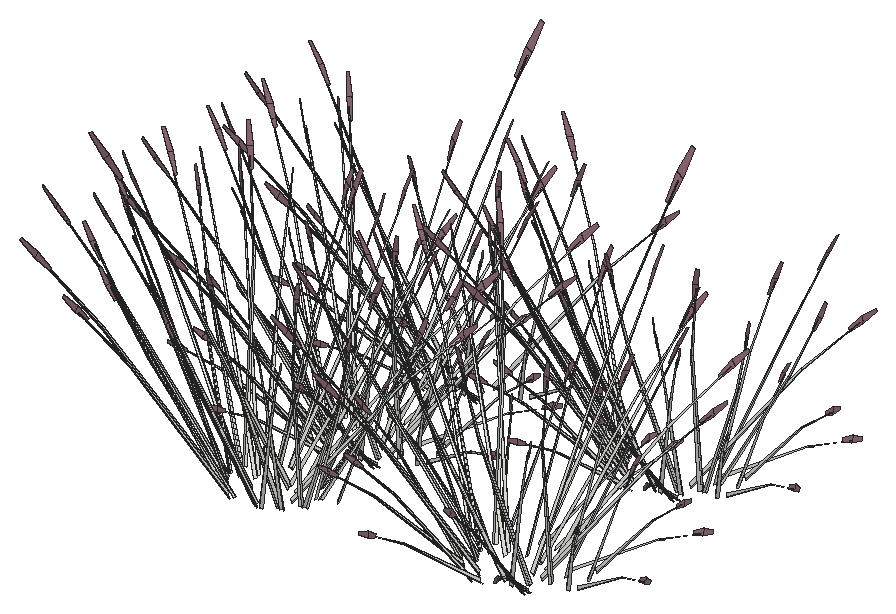
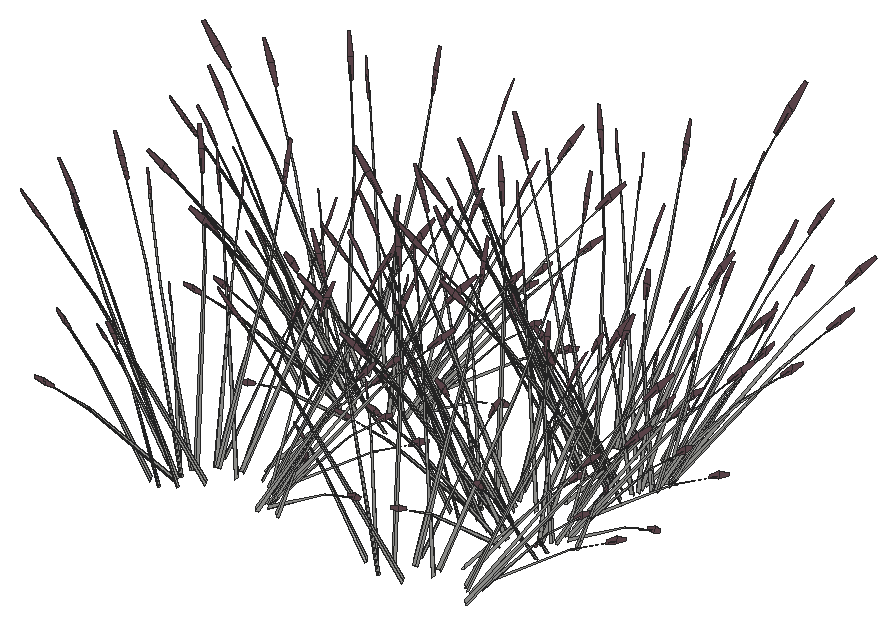
# SketchUp Ruby script. Lengths in inches.
U = 1.inch
M = Sketchup.active_model
def pt(a) = Geom::Point3d.new(a.map { |v| v * U })
def face(e, loops, mat)
  f = e.add_face(loops[0].map { |a| pt(a) })
  loops[1..].each { |l| e.add_face(l.map { |a| pt(a) }).erase! }
  f.material = f.back_material = mat if mat
  f
end
# faces: each face lists its corners as indices into pts; further lists are holes
def faces(e, pts, list, mat = nil) = list.each { |f| face(e, (f[0].is_a?(Array) ? f : [f]).map { |l| l.map { |i| pts[i] } }, mat) }
# xy, xz, yz: faces in a plane at the given z, y or x. An outline is a flat list of corners, or four numbers for a rectangle; further outlines are holes
def ring(l) = l.size == 4 ? [[l[0], l[1]], [l[2], l[1]], [l[2], l[3]], [l[0], l[3]]] : l.each_slice(2).to_a
def flat(e, list, mat, &to3) = list.each { |f| face(e, (f[0].is_a?(Array) ? f : [f]).map { |l| ring(l).map { |u, v| to3.(u, v) } }, mat) }
def xy(e, z, list, mat = nil) = flat(e, list, mat) { |x, y| [x, y, z] }
def xz(e, y, list, mat = nil) = flat(e, list, mat) { |x, z| [x, y, z] }
def yz(e, x, list, mat = nil) = flat(e, list, mat) { |y, z| [x, y, z] }
def lines(e, pts, list) = list.each { |a, b| e.add_line(pt(pts[a]), pt(pts[b])) }
# prism: a flat outline (further loops are holes) pulled along v
def prism(e, loops, v, mat = nil)
  f = face(e, loops, mat); d = Geom::Vector3d.new(v.map { |x| x * U })
  f.pushpull(f.normal.samedirection?(d) ? d.length : -d.length)
end
def box(e, o, s, mat = nil) = prism(e, [[o, [o[0] + s[0], o[1], o[2]], [o[0] + s[0], o[1] + s[1], o[2]], [o[0], o[1] + s[1], o[2]]]], [0, 0, s[2]], mat)
def at(x, y, z, deg = 0) = Geom::Transformation.translation(pt([x, y, z])) * Geom::Transformation.rotation(ORIGIN, Z_AXIS, deg.degrees)
def axes(o, x, y, z) = Geom::Transformation.new([*x, 0, *y, 0, *z, 0, *pt(o).to_a, 1])
def part(name) = M.definitions.add(name)
# library, detail: a bought-in or finely detailed component or shape, given as its bounding box
def library(name, o, s) = part(name).tap { |d| box(d.entities, o, s) }
def detail(e, o, s) = box(e.add_group.entities, o, s)
def put(e, d, t, mat = nil) = e.add_instance(d, t).tap { |i| i.material = mat if mat }
def group(e, t, mat = nil) = e.add_group.tap { |g| g.transformation = t; g.material = mat if mat }.entities
root = M.entities
M.materials.add("LightPink_Translucent").color = [144, 107, 117]
c1 = part("blade")
p = [[2.15,0.21,22],[0,0.17,0],[0.09,0.45,0],[2.18,0.31,22],[2.29,0.31,22],[0.38,0.45,0],
  [2.48,0.24,33],[2.49,0.24,33],[2.48,0.22,33]]
faces(c1.entities,p,[[0,1,2,3],[4,5,2,3],[6,3,4,7],[8,0,3,6]])
c2 = part("seeds")
p = [[0.3,-0.1,1.38],[-0.01,-0.03,1.59],[-0.01,-0.03,0.03],[0.14,-0.07,-0.07],[0.29,-0.03,3],[0.15,0.01,3.11]]
faces(c2.entities,p,[[0,1,2,3],[1,0,4,5]],"LightPink_Translucent")
c3 = part("blade with seeds")
put(c3.entities,c1,at(0,0,0))
put(c3.entities,c2,axes([2.4,0.25,30.99],[1.5799,-0.05474,1.17369],[-0.12525,1.92788,0.29478],[-0.07173,-0.02425,1.56792]))
put(root,c3,axes([27.78,17.96,46.13],[0.28013,0.33252,1.71376],[-1.29445,0.27994,0.13857],[-0.29256,-0.52202,0.73262]))
put(root,c3,axes([31.34,17.49,46.78],[0.36946,-0.79643,-0.35414],[1.07787,0.23229,0.4572],[-0.09883,-0.32066,0.87481]))
put(root,c3,axes([32.15,18.55,46.13],[-0.22818,0.35597,1.71376],[-0.95725,-0.73667,0.13857],[0.43183,-0.45914,0.73262]))
put(root,c3,axes([31.82,18,47.29],[-1.19922,0.48218,-0.1216],[-0.58932,-0.85579,-0.67495],[-0.15822,-0.36063,1.02557]))
put(root,c3,axes([34.3125,19.08,47.29],[-1.34686,-0.05131,-0.1216],[0.03681,-0.97156,-0.67495],[0.09356,-0.37418,1.02557]))
put(root,c3,axes([34.22,18.46,46.78],[0.82919,-0.54528,-0.35414],[0.78493,0.62262,0.4572],[0.11943,-0.31634,0.87481]))
put(root,c3,axes([28.23,17.78,46.78],[-0.18927,-0.83419,-0.35414],[1.08199,-0.22027,0.4572],[-0.29062,-0.23905,0.87481]))
put(root,c3,axes([60.8,22.02,45.875],[0.28013,0.33252,1.71376],[-1.29445,0.27994,0.13857],[-0.29256,-0.52202,0.73262]))
put(root,c3,axes([25.9,19,46.13],[0.45521,0.17844,1.71376],[-0.94204,0.74856,0.13857],[-0.58713,-0.33769,0.73262]))
put(root,c3,axes([62.93,19.82,46.72],[-0.18744,-0.14521,1.74944],[-1.25089,0.09206,-0.27667],[-0.19964,-0.34731,0.14031]))
put(root,c3,axes([68.55,21.6,46.72],[-0.01183,-0.20612,1.74944],[-0.99913,-0.59572,-0.27667],[0.15447,-0.36112,0.14031]))
put(root,c3,axes([65.17,22.61,45.875],[-0.22818,0.35597,1.71376],[-0.95725,-0.73667,0.13857],[0.43183,-0.45914,0.73262]))
put(root,c3,axes([68.29,20.86,46.71],[-0.12446,0.07911,1.77383],[-1.21937,-0.26689,-0.16761],[-0.04414,-0.34521,0.31391]))
put(root,c3,axes([35.78,20.99,47.29],[-1.1336,-0.57106,-0.1216],[0.65308,-0.827,-0.67495],[0.32027,-0.28747,1.02557]))
put(root,c3,axes([31.1,24.11,45.58],[1.05902,0.41762,1.51261],[-1.03748,0.89969,0.59816],[-0.46471,-0.53324,1.26806]))
put(root,c3,axes([61.65,19.34,46.71],[-0.02286,0.12414,1.77383],[-1.12758,0.45052,-0.16761],[-0.33182,-0.23029,0.31391]))
put(root,c3,axes([64.84,22.06,47.03],[-1.19922,0.48218,-0.1216],[-0.58932,-0.85579,-0.67495],[-0.15822,-0.36063,1.02557]))
put(root,c3,axes([67.33,23.14,47.03],[-1.34686,-0.05131,-0.1216],[0.03681,-0.97156,-0.67495],[0.09356,-0.37418,1.02557]))
put(root,c3,axes([36.1,20.41,46.78],[1.06674,-0.14801,-0.35414],[0.28168,0.84611,0.4572],[0.30569,-0.22726,0.87481]))
put(root,c3,axes([25.73,19.25,46.78],[-0.69728,-0.64842,-0.35414],[0.79619,-0.61382,0.4572],[-0.40453,-0.09339,0.87481]))
put(root,c3,axes([58.92,23.06,45.875],[0.45521,0.17844,1.71376],[-0.94204,0.74856,0.13857],[-0.58713,-0.33769,0.73262]))
put(root,c3,axes([58.83,21.41,46.72],[-0.26368,-0.00731,1.74944],[-0.83946,0.73103,-0.27667],[-0.44791,-0.14937,0.14031]))
put(root,c3,axes([68.79,25.05,47.03],[-1.1336,-0.57106,-0.1216],[0.65308,-0.827,-0.67495],[0.32027,-0.28747,1.02557]))
put(root,c3,axes([26.53,19.18,47.29],[-0.06562,1.05324,-0.1216],[-1.2424,-0.02879,-0.67495],[-0.4785,-0.07316,1.02557]))
put(root,c3,axes([35.82,23.22,47.29],[-0.6166,-0.93779,-0.1216],[1.09436,-0.46085,-0.67495],[0.46117,-0.12373,1.02557]))
put(root,c3,axes([71.59,24.8,46.71],[-0.16006,-0.00787,1.77383],[-0.66468,-0.8428,-0.16761],[0.26693,-0.27711,0.31391]))
put(root,c3,axes([24.94,20.63,46.13],[0.50831,-0.02346,1.71376],[-0.33721,1.01661,0.13857],[-0.72439,-0.06288,0.73262]))
put(root,c3,axes([36.47,22.84,46.78],[1.01846,0.28891,-0.35414],[-0.29705,0.84289,0.4572],[0.41005,-0.07729,0.87481]))
put(root,c3,axes([72.1875,25.8125,46.72],[0.17006,-0.15775,1.74944],[-0.21766,-0.96766,-0.27667],[0.42669,-0.18347,0.14031]))
put(root,c3,axes([24.5,21.5,46.78],[-1.01846,-0.28891,-0.35414],[0.29705,-0.84289,0.4572],[-0.41005,0.07729,0.87481]))
put(root,c3,axes([57.82,22.03,46.71],[0.09085,0.10335,1.77383],[-0.43798,0.92907,-0.16761],[-0.44357,0.00672,0.31391]))
put(root,c3,axes([33.69,21.8,46.13],[-0.50831,0.02346,1.71376],[0.33721,-1.01661,0.13857],[0.72439,0.06288,0.73262]))
put(root,c3,axes([59.54,23.24,47.03],[-0.06562,1.05324,-0.1216],[-1.2424,-0.02879,-0.67495],[-0.4785,-0.07316,1.02557]))
put(root,c3,axes([68.84,27.28,47.03],[-0.6166,-0.93779,-0.1216],[1.09436,-0.46085,-0.67495],[0.46117,-0.12373,1.02557]))
put(root,c3,axes([57.96,24.69,45.875],[0.50831,-0.02346,1.71376],[-0.33721,1.01661,0.13857],[-0.72439,-0.06288,0.73262]))
put(root,c3,axes([27.6,21.36,45.59],[0.34834,-0.14982,1.77064],[0.12012,1.04605,0.13857],[-0.75452,0.1388,0.63284]))
put(root,c3,axes([25.14,21.125,47.29],[0.6166,0.93779,-0.1216],[-1.09436,0.46085,-0.67495],[-0.46117,0.12373,1.02557]))
put(root,c3,axes([37.3125,25.19,46.18],[-0.23455,-0.87059,-0.03492],[1.10861,-0.20015,-0.15832],[0.23151,0.05519,0.52218]))
put(root,c3,axes([34.4375,25.17,47.29],[0.06562,-1.05324,-0.1216],[1.2424,0.02879,-0.67495],[0.4785,0.07316,1.02557]))
put(root,c3,axes([29.33,34.02,45.875],[0.28013,0.33252,1.71376],[-1.29445,0.27994,0.13857],[-0.29256,-0.52202,0.73262]))
put(root,c3,axes([31.46,31.82,46.72],[-0.18744,-0.14521,1.74944],[-1.25089,0.09206,-0.27667],[-0.19964,-0.34731,0.14031]))
put(root,c3,axes([25.16,22.42,46.13],[0.42521,-0.21906,1.71376],[0.35798,1.01226,0.13857],[-0.66754,0.22878,0.73262]))
put(root,c3,axes([37.08,33.6,46.72],[-0.01183,-0.20612,1.74944],[-0.99913,-0.59572,-0.27667],[0.15447,-0.36112,0.14031]))
put(root,c3,axes([33.7,34.61,45.875],[-0.22818,0.35597,1.71376],[-0.95725,-0.73667,0.13857],[0.43183,-0.45914,0.73262]))
put(root,c3,axes([36.81,32.86,46.71],[-0.12446,0.07911,1.77383],[-1.21937,-0.26689,-0.16761],[-0.04414,-0.34521,0.31391]))
put(root,c3,axes([66.71,25.86,45.875],[-0.50831,0.02346,1.71376],[0.33721,-1.01661,0.13857],[0.72439,0.06288,0.73262]))
put(root,c3,axes([30.18,31.34,46.71],[-0.02286,0.12414,1.77383],[-1.12758,0.45052,-0.16761],[-0.33182,-0.23029,0.31391]))
put(root,c3,axes([35.24,25.1,46.78],[0.69728,0.64842,-0.35414],[-0.79619,0.61382,0.4572],[0.40453,0.09339,0.87481]))
put(root,c3,axes([33.37,34.06,47.03],[-1.19922,0.48218,-0.1216],[-0.58932,-0.85579,-0.67495],[-0.15822,-0.36063,1.02557]))
put(root,c3,axes([24.87,23.93,46.78],[-1.06674,0.14801,-0.35414],[-0.28168,-0.84611,0.4572],[-0.30569,0.22726,0.87481]))
put(root,c3,axes([35.86,35.14,47.03],[-1.34686,-0.05131,-0.1216],[0.03681,-0.97156,-0.67495],[0.09356,-0.37418,1.02557]))
put(root,c3,axes([71.29,30.07,46.71],[-0.11081,-0.09067,1.77383],[0.2424,-0.97188,-0.16761],[0.43649,-0.06209,0.31391]))
put(root,c3,axes([56.87,26.125,46.72],[-0.20012,0.13446,1.74944],[0.01702,0.98243,-0.27667],[-0.45871,0.12776,0.14031]))
put(root,c3,axes([58.16,25.1875,47.03],[0.6166,0.93779,-0.1216],[-1.09436,0.46085,-0.67495],[-0.46117,0.12373,1.02557]))
put(root,c3,axes([70.33,29.26,45.93],[-0.23455,-0.87059,-0.03492],[1.10861,-0.20015,-0.15832],[0.23151,0.05519,0.52218]))
put(root,c3,axes([67.46,29.23,47.03],[0.06562,-1.05324,-0.1216],[1.2424,0.02879,-0.67495],[0.4785,0.07316,1.02557]))
put(root,c3,axes([32.73,23.43,46.13],[-0.45521,-0.17844,1.71376],[0.94204,-0.74856,0.13857],[0.58713,0.33769,0.73262]))
put(root,c3,axes([27.45,35.06,45.875],[0.45521,0.17844,1.71376],[-0.94204,0.74856,0.13857],[-0.58713,-0.33769,0.73262]))
put(root,c3,axes([25.1875,23.36,47.29],[1.1336,0.57106,-0.1216],[-0.65308,0.827,-0.67495],[-0.32027,0.28747,1.02557]))
put(root,c3,axes([31.99,26.31,47.29],[0.73026,-0.88648,-0.1216],[1.05755,0.51071,-0.67495],[0.36761,0.25045,1.02557]))
put(root,c3,axes([26.71,23.1,46.13],[0.30609,-0.31822,1.71376],[0.77286,0.85893,0.13857],[-0.53009,0.39116,0.73262]))
put(root,c3,axes([68.54,28.6,46.72],[0.26289,-0.01751,1.74944],[0.72108,-0.8046,-0.27667],[0.46761,0.10621,0.14031]))
put(root,c3,axes([58.17,26.48,45.875],[0.42521,-0.21906,1.71376],[0.35798,1.01226,0.13857],[-0.66754,0.22878,0.73262]))
put(root,c3,axes([27.36,33.41,46.72],[-0.26368,-0.00731,1.74944],[-0.83946,0.73103,-0.27667],[-0.44791,-0.14937,0.14031]))
put(root,c3,axes([37.32,37.05,47.03],[-1.1336,-0.57106,-0.1216],[0.65308,-0.827,-0.67495],[0.32027,-0.28747,1.02557]))
put(root,c3,axes([40.11,36.8,46.71],[-0.16006,-0.00787,1.77383],[-0.66468,-0.8428,-0.16761],[0.26693,-0.27711,0.31391]))
put(root,c3,axes([54.65,27.12,46.71],[0.1564,0.02778,1.77383],[0.48382,0.91506,-0.16761],[-0.32016,0.24017,0.31391]))
put(root,c3,axes([26.48,23.88,46.13],[0.22818,-0.35597,1.71376],[0.95725,0.73667,0.13857],[-0.43183,0.45914,0.73262]))
put(root,c3,axes([26.75,25.89,46.78],[-0.82919,0.54528,-0.35414],[-0.78493,-0.62262,0.4572],[-0.11943,0.31634,0.87481]))
put(root,c3,axes([29.14,26.35,47.29],[1.19922,-0.48218,-0.1216],[0.58932,0.85579,-0.67495],[0.15822,0.36063,1.02557]))
put(root,c3,axes([65.75,27.49,45.875],[-0.45521,-0.17844,1.71376],[0.94204,-0.74856,0.13857],[0.58713,0.33769,0.73262]))
put(root,c3,axes([65.84,25.14,46.47],[-1.05895,-0.53811,1.38283],[1.11816,-0.83781,0.59665],[0.34166,0.5049,1.33663]))
put(root,c3,axes([30.86,24.47,46.13],[-0.28013,-0.33252,1.71376],[1.29445,-0.27994,0.13857],[0.29256,0.52202,0.73262]))
put(root,c3,axes([58.2,27.42,47.03],[1.1336,0.57106,-0.1216],[-0.65308,0.827,-0.67495],[-0.32027,0.28747,1.02557]))
put(root,c3,axes([65.01,30.375,47.03],[0.73026,-0.88648,-0.1216],[1.05755,0.51071,-0.67495],[0.36761,0.25045,1.02557]))
put(root,c3,axes([29.625,26.85,46.78],[-0.36946,0.79643,-0.35414],[-1.07787,-0.23229,0.4572],[0.09883,0.32066,0.87481]))
put(root,c3,axes([59.73,27.16,45.875],[0.30609,-0.31822,1.71376],[0.77286,0.85893,0.13857],[-0.53009,0.39116,0.73262]))
put(root,c3,axes([40.72,37.8125,46.72],[0.17006,-0.15775,1.74944],[-0.21766,-0.96766,-0.27667],[0.42669,-0.18347,0.14031]))
put(root,c3,axes([28.57,24.64,46.13],[-0.02999,-0.3975,1.71376],[1.30002,0.26369,0.13857],[-0.08041,0.56647,0.73262]))
put(root,c3,axes([64.05,31.11,46.71],[0.00363,-0.12539,1.77383],[1.0502,-0.55319,-0.16761],[0.36479,0.19745,0.31391]))
put(root,c3,axes([26.35,34.03,46.71],[0.09085,0.10335,1.77383],[-0.43798,0.92907,-0.16761],[-0.44357,0.00672,0.31391]))
put(root,c3,axes([28.07,35.24,47.03],[-0.06562,1.05324,-0.1216],[-1.2424,-0.02879,-0.67495],[-0.4785,-0.07316,1.02557]))
put(root,c3,axes([37.37,39.28,47.03],[-0.6166,-0.93779,-0.1216],[1.09436,-0.46085,-0.67495],[0.46117,-0.12373,1.02557]))
put(root,c3,axes([26.49,36.69,45.875],[0.50831,-0.02346,1.71376],[-0.33721,1.01661,0.13857],[-0.72439,-0.06288,0.73262]))
put(root,c3,axes([59.5,27.95,45.875],[0.22818,-0.35597,1.71376],[0.95725,0.73667,0.13857],[-0.43183,0.45914,0.73262]))
put(root,c3,axes([26.85,26.66,45.61],[0.02693,-0.53464,1.54345],[1.21102,0.2824,0.21329],[-0.10493,0.5698,0.72882]))
put(root,c3,axes([56.9,29.79,46.72],[-0.03046,0.20495,1.74944],[0.86449,0.71297,-0.27667],[-0.22632,0.33716,0.14031]))
put(root,c3,axes([62.16,30.41,47.03],[1.19922,-0.48218,-0.1216],[0.58932,0.85579,-0.67495],[0.15822,0.36063,1.02557]))
put(root,c3,axes([63.875,28.53,45.875],[-0.28013,-0.33252,1.71376],[1.29445,-0.27994,0.13857],[0.29256,0.52202,0.73262]))
put(root,c3,axes([56.81,31.89,46.71],[0.13903,-0.06253,1.77383],[1.14912,0.41591,-0.16761],[-0.027,0.34629,0.31391]))
put(root,c3,axes([61.59,28.7,45.875],[-0.02999,-0.3975,1.71376],[1.30002,0.26369,0.13857],[-0.08041,0.56647,0.73262]))
put(root,c3,axes([35.24,37.86,45.875],[-0.50831,0.02346,1.71376],[0.33721,-1.01661,0.13857],[0.72439,0.06288,0.73262]))
put(root,c3,axes([61.88,32.33,46.72],[0.15534,0.16677,1.74944],[1.25362,0.06552,-0.27667],[0.12606,0.3678,0.14031]))
put(root,c3,axes([60.59,49.31,45.875],[0.28013,0.33252,1.71376],[-1.29445,0.27994,0.13857],[-0.29256,-0.52202,0.73262]))
put(root,c3,axes([39.82,42.07,46.71],[-0.11081,-0.09067,1.77383],[0.2424,-0.97188,-0.16761],[0.43649,-0.06209,0.31391]))
put(root,c3,axes([62.73,47.1,46.72],[-0.18744,-0.14521,1.74944],[-1.25089,0.09206,-0.27667],[-0.19964,-0.34731,0.14031]))
put(root,c3,axes([25.4,38.125,46.72],[-0.20012,0.13446,1.74944],[0.01702,0.98243,-0.27667],[-0.45871,0.12776,0.14031]))
put(root,c3,axes([26.69,37.1875,47.03],[0.6166,0.93779,-0.1216],[-1.09436,0.46085,-0.67495],[-0.46117,0.12373,1.02557]))
put(root,c3,axes([38.86,41.26,45.93],[-0.23455,-0.87059,-0.03492],[1.10861,-0.20015,-0.15832],[0.23151,0.05519,0.52218]))
put(root,c3,axes([35.98,41.23,47.03],[0.06562,-1.05324,-0.1216],[1.2424,0.02879,-0.67495],[0.4785,0.07316,1.02557]))
put(root,c3,axes([68.35,48.88,46.72],[-0.01183,-0.20612,1.74944],[-0.99913,-0.59572,-0.27667],[0.15447,-0.36112,0.14031]))
put(root,c3,axes([64.15,48.84,46.53],[0.36946,-0.79643,-0.35414],[1.07787,0.23229,0.4572],[-0.09883,-0.32066,0.87481]))
put(root,c3,axes([64.96,49.89,45.875],[-0.22818,0.35597,1.71376],[-0.95725,-0.73667,0.13857],[0.43183,-0.45914,0.73262]))
put(root,c3,axes([68.08,48.14,46.71],[-0.12446,0.07911,1.77383],[-1.21937,-0.26689,-0.16761],[-0.04414,-0.34521,0.31391]))
put(root,c3,axes([37.0625,40.6,46.72],[0.26289,-0.01751,1.74944],[0.72108,-0.8046,-0.27667],[0.46761,0.10621,0.14031]))
put(root,c3,axes([26.7,38.48,45.875],[0.42521,-0.21906,1.71376],[0.35798,1.01226,0.13857],[-0.66754,0.22878,0.73262]))
put(root,c3,axes([61.44,46.625,46.71],[-0.02286,0.12414,1.77383],[-1.12758,0.45052,-0.16761],[-0.33182,-0.23029,0.31391]))
put(root,c3,axes([64.63,49.34,47.03],[-1.19922,0.48218,-0.1216],[-0.58932,-0.85579,-0.67495],[-0.15822,-0.36063,1.02557]))
put(root,c3,axes([67.12,50.43,47.03],[-1.34686,-0.05131,-0.1216],[0.03681,-0.97156,-0.67495],[0.09356,-0.37418,1.02557]))
put(root,c3,axes([67.03,49.8,46.53],[0.82919,-0.54528,-0.35414],[0.78493,0.62262,0.4572],[0.11943,-0.31634,0.87481]))
put(root,c3,axes([61.04,49.13,46.53],[-0.18927,-0.83419,-0.35414],[1.08199,-0.22027,0.4572],[-0.29062,-0.23905,0.87481]))
put(root,c3,axes([23.18,39.12,46.71],[0.1564,0.02778,1.77383],[0.48382,0.91506,-0.16761],[-0.32016,0.24017,0.31391]))
put(root,c3,axes([29.03,53.05,45.875],[0.28013,0.33252,1.71376],[-1.29445,0.27994,0.13857],[-0.29256,-0.52202,0.73262]))
put(root,c3,axes([31.16,50.85,46.72],[-0.18744,-0.14521,1.74944],[-1.25089,0.09206,-0.27667],[-0.19964,-0.34731,0.14031]))
put(root,c3,axes([58.71,50.34,45.875],[0.45521,0.17844,1.71376],[-0.94204,0.74856,0.13857],[-0.58713,-0.33769,0.73262]))
put(root,c3,axes([34.28,39.49,45.875],[-0.45521,-0.17844,1.71376],[0.94204,-0.74856,0.13857],[0.58713,0.33769,0.73262]))
put(root,c3,axes([34.36,37.14,46.47],[-1.05895,-0.53811,1.38283],[1.11816,-0.83781,0.59665],[0.34166,0.5049,1.33663]))
put(root,c3,axes([26.73,39.42,47.03],[1.1336,0.57106,-0.1216],[-0.65308,0.827,-0.67495],[-0.32027,0.28747,1.02557]))
put(root,c3,axes([36.78,52.625,46.72],[-0.01183,-0.20612,1.74944],[-0.99913,-0.59572,-0.27667],[0.15447,-0.36112,0.14031]))
put(root,c3,axes([33.4,53.64,45.875],[-0.22818,0.35597,1.71376],[-0.95725,-0.73667,0.13857],[0.43183,-0.45914,0.73262]))
put(root,c3,axes([36.52,51.89,46.71],[-0.12446,0.07911,1.77383],[-1.21937,-0.26689,-0.16761],[-0.04414,-0.34521,0.31391]))
put(root,c3,axes([33.54,42.375,47.03],[0.73026,-0.88648,-0.1216],[1.05755,0.51071,-0.67495],[0.36761,0.25045,1.02557]))
put(root,c3,axes([28.26,39.16,45.875],[0.30609,-0.31822,1.71376],[0.77286,0.85893,0.13857],[-0.53009,0.39116,0.73262]))
put(root,c3,axes([58.625,48.7,46.72],[-0.26368,-0.00731,1.74944],[-0.83946,0.73103,-0.27667],[-0.44791,-0.14937,0.14031]))
put(root,c3,axes([68.59,52.34,47.03],[-1.1336,-0.57106,-0.1216],[0.65308,-0.827,-0.67495],[0.32027,-0.28747,1.02557]))
put(root,c3,axes([32.58,43.11,46.71],[0.00363,-0.12539,1.77383],[1.0502,-0.55319,-0.16761],[0.36479,0.19745,0.31391]))
put(root,c3,axes([29.88,50.37,46.71],[-0.02286,0.12414,1.77383],[-1.12758,0.45052,-0.16761],[-0.33182,-0.23029,0.31391]))
put(root,c3,axes([71.38,52.09,46.71],[-0.16006,-0.00787,1.77383],[-0.66468,-0.8428,-0.16761],[0.26693,-0.27711,0.31391]))
put(root,c3,axes([33.07,53.09,47.03],[-1.19922,0.48218,-0.1216],[-0.58932,-0.85579,-0.67495],[-0.15822,-0.36063,1.02557]))
put(root,c3,axes([35.56,54.17,47.03],[-1.34686,-0.05131,-0.1216],[0.03681,-0.97156,-0.67495],[0.09356,-0.37418,1.02557]))
put(root,c3,axes([68.9,51.76,46.53],[1.06674,-0.14801,-0.35414],[0.28168,0.84611,0.4572],[0.30569,-0.22726,0.87481]))
put(root,c3,axes([58.54,50.6,46.53],[-0.69728,-0.64842,-0.35414],[0.79619,-0.61382,0.4572],[-0.40453,-0.09339,0.87481]))
put(root,c3,axes([28.03,39.95,45.875],[0.22818,-0.35597,1.71376],[0.95725,0.73667,0.13857],[-0.43183,0.45914,0.73262]))
put(root,c3,axes([25.43,41.79,46.72],[-0.03046,0.20495,1.74944],[0.86449,0.71297,-0.27667],[-0.22632,0.33716,0.14031]))
put(root,c3,axes([27.15,54.09,45.875],[0.45521,0.17844,1.71376],[-0.94204,0.74856,0.13857],[-0.58713,-0.33769,0.73262]))
put(root,c3,axes([30.6875,42.41,47.03],[1.19922,-0.48218,-0.1216],[0.58932,0.85579,-0.67495],[0.15822,0.36063,1.02557]))
put(root,c3,axes([71.98,53.1,46.72],[0.17006,-0.15775,1.74944],[-0.21766,-0.96766,-0.27667],[0.42669,-0.18347,0.14031]))
put(root,c3,axes([32.4,40.53,45.875],[-0.28013,-0.33252,1.71376],[1.29445,-0.27994,0.13857],[0.29256,0.52202,0.73262]))
put(root,c3,axes([57.61,49.32,46.71],[0.09085,0.10335,1.77383],[-0.43798,0.92907,-0.16761],[-0.44357,0.00672,0.31391]))
put(root,c3,axes([27.0625,52.44,46.72],[-0.26368,-0.00731,1.74944],[-0.83946,0.73103,-0.27667],[-0.44791,-0.14937,0.14031]))
put(root,c3,axes([37.02,56.08,47.03],[-1.1336,-0.57106,-0.1216],[0.65308,-0.827,-0.67495],[0.32027,-0.28747,1.02557]))
put(root,c3,axes([25.33,43.89,46.71],[0.13903,-0.06253,1.77383],[1.14912,0.41591,-0.16761],[-0.027,0.34629,0.31391]))
put(root,c3,axes([30.11,40.7,45.875],[-0.02999,-0.3975,1.71376],[1.30002,0.26369,0.13857],[-0.08041,0.56647,0.73262]))
put(root,c3,axes([39.82,55.83,46.71],[-0.16006,-0.00787,1.77383],[-0.66468,-0.8428,-0.16761],[0.26693,-0.27711,0.31391]))
put(root,c3,axes([59.33,50.52,47.03],[-0.06562,1.05324,-0.1216],[-1.2424,-0.02879,-0.67495],[-0.4785,-0.07316,1.02557]))
put(root,c3,axes([68.63,54.57,47.03],[-0.6166,-0.93779,-0.1216],[1.09436,-0.46085,-0.67495],[0.46117,-0.12373,1.02557]))
put(root,c3,axes([57.75,51.98,45.875],[0.50831,-0.02346,1.71376],[-0.33721,1.01661,0.13857],[-0.72439,-0.06288,0.73262]))
put(root,c3,axes([30.41,44.33,46.72],[0.15534,0.16677,1.74944],[1.25362,0.06552,-0.27667],[0.12606,0.3678,0.14031]))
put(root,c3,axes([40.42,56.84,46.72],[0.17006,-0.15775,1.74944],[-0.21766,-0.96766,-0.27667],[0.42669,-0.18347,0.14031]))
put(root,c3,axes([69.28,54.19,46.53],[1.01846,0.28891,-0.35414],[-0.29705,0.84289,0.4572],[0.41005,-0.07729,0.87481]))
put(root,c3,axes([26.05,53.0625,46.71],[0.09085,0.10335,1.77383],[-0.43798,0.92907,-0.16761],[-0.44357,0.00672,0.31391]))
put(root,c3,axes([57.31,52.85,46.53],[-1.01846,-0.28891,-0.35414],[0.29705,-0.84289,0.4572],[-0.41005,0.07729,0.87481]))
put(root,c3,axes([66.5,53.15,45.875],[-0.50831,0.02346,1.71376],[0.33721,-1.01661,0.13857],[0.72439,0.06288,0.73262]))
put(root,c3,axes([27.77,54.27,47.03],[-0.06562,1.05324,-0.1216],[-1.2424,-0.02879,-0.67495],[-0.4785,-0.07316,1.02557]))
put(root,c3,axes([37.07,58.3125,47.03],[-0.6166,-0.93779,-0.1216],[1.09436,-0.46085,-0.67495],[0.46117,-0.12373,1.02557]))
put(root,c3,axes([26.19,55.72,45.875],[0.50831,-0.02346,1.71376],[-0.33721,1.01661,0.13857],[-0.72439,-0.06288,0.73262]))
put(root,c3,axes([71.08,57.35,46.71],[-0.11081,-0.09067,1.77383],[0.2424,-0.97188,-0.16761],[0.43649,-0.06209,0.31391]))
put(root,c3,axes([56.66,53.41,46.72],[-0.20012,0.13446,1.74944],[0.01702,0.98243,-0.27667],[-0.45871,0.12776,0.14031]))
put(root,c3,axes([57.95,52.47,47.03],[0.6166,0.93779,-0.1216],[-1.09436,0.46085,-0.67495],[-0.46117,0.12373,1.02557]))
put(root,c3,axes([70.12,56.54,45.93],[-0.23455,-0.87059,-0.03492],[1.10861,-0.20015,-0.15832],[0.23151,0.05519,0.52218]))
put(root,c3,axes([67.25,56.52,47.03],[0.06562,-1.05324,-0.1216],[1.2424,0.02879,-0.67495],[0.4785,0.07316,1.02557]))
put(root,c3,axes([68.33,55.88,46.72],[0.26289,-0.01751,1.74944],[0.72108,-0.8046,-0.27667],[0.46761,0.10621,0.14031]))
put(root,c3,axes([57.96,53.76,45.875],[0.42521,-0.21906,1.71376],[0.35798,1.01226,0.13857],[-0.66754,0.22878,0.73262]))
put(root,c3,axes([34.9375,56.89,45.875],[-0.50831,0.02346,1.71376],[0.33721,-1.01661,0.13857],[0.72439,0.06288,0.73262]))
put(root,c3,axes([54.4375,54.4,46.71],[0.1564,0.02778,1.77383],[0.48382,0.91506,-0.16761],[-0.32016,0.24017,0.31391]))
